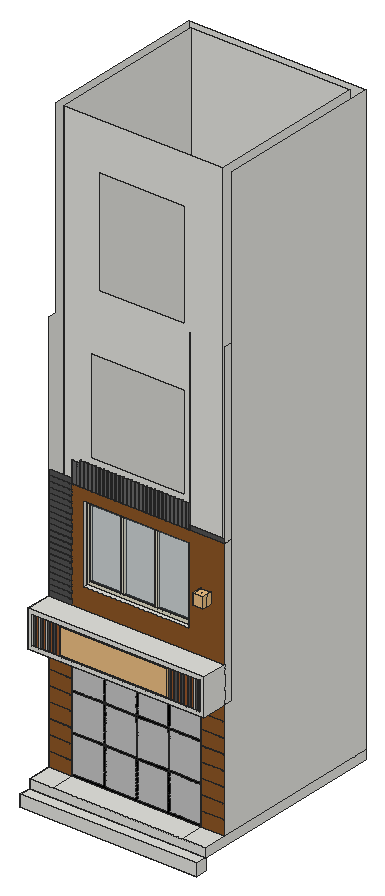
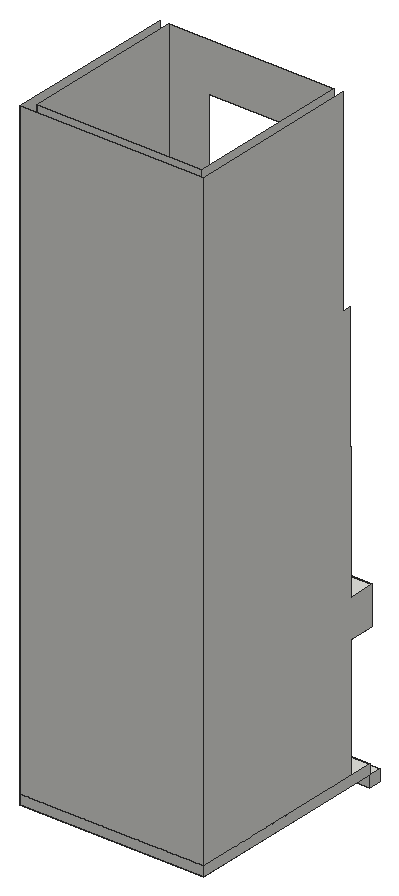
# SketchUp Ruby script. Lengths in inches.
U = 1.inch
M = Sketchup.active_model
def pt(a) = Geom::Point3d.new(a.map { |v| v * U })
def face(e, loops, mat)
  f = e.add_face(loops[0].map { |a| pt(a) })
  loops[1..].each { |l| e.add_face(l.map { |a| pt(a) }).erase! }
  f.material = f.back_material = mat if mat
  f
end
# faces: each face lists its corners as indices into pts; further lists are holes
def faces(e, pts, list, mat = nil) = list.each { |f| face(e, (f[0].is_a?(Array) ? f : [f]).map { |l| l.map { |i| pts[i] } }, mat) }
# xy, xz, yz: faces in a plane at the given z, y or x. An outline is a flat list of corners, or four numbers for a rectangle; further outlines are holes
def ring(l) = l.size == 4 ? [[l[0], l[1]], [l[2], l[1]], [l[2], l[3]], [l[0], l[3]]] : l.each_slice(2).to_a
def flat(e, list, mat, &to3) = list.each { |f| face(e, (f[0].is_a?(Array) ? f : [f]).map { |l| ring(l).map { |u, v| to3.(u, v) } }, mat) }
def xy(e, z, list, mat = nil) = flat(e, list, mat) { |x, y| [x, y, z] }
def xz(e, y, list, mat = nil) = flat(e, list, mat) { |x, z| [x, y, z] }
def yz(e, x, list, mat = nil) = flat(e, list, mat) { |y, z| [x, y, z] }
def lines(e, pts, list) = list.each { |a, b| e.add_line(pt(pts[a]), pt(pts[b])) }
# prism: a flat outline (further loops are holes) pulled along v
def prism(e, loops, v, mat = nil)
  f = face(e, loops, mat); d = Geom::Vector3d.new(v.map { |x| x * U })
  f.pushpull(f.normal.samedirection?(d) ? d.length : -d.length)
end
def box(e, o, s, mat = nil) = prism(e, [[o, [o[0] + s[0], o[1], o[2]], [o[0] + s[0], o[1] + s[1], o[2]], [o[0], o[1] + s[1], o[2]]]], [0, 0, s[2]], mat)
def at(x, y, z, deg = 0) = Geom::Transformation.translation(pt([x, y, z])) * Geom::Transformation.rotation(ORIGIN, Z_AXIS, deg.degrees)
def axes(o, x, y, z) = Geom::Transformation.new([*x, 0, *y, 0, *z, 0, *pt(o).to_a, 1])
def part(name) = M.definitions.add(name)
# library, detail: a bought-in or finely detailed component or shape, given as its bounding box
def library(name, o, s) = part(name).tap { |d| box(d.entities, o, s) }
def detail(e, o, s) = box(e.add_group.entities, o, s)
def put(e, d, t, mat = nil) = e.add_instance(d, t).tap { |i| i.material = mat if mat }
def group(e, t, mat = nil) = e.add_group.tap { |g| g.transformation = t; g.material = mat if mat }.entities
root = M.entities
M.materials.add("Glass").color = [171, 209, 242]
M.materials["Glass"].alpha = 0.09
M.materials.add("Plastic_SSS_01_White").color = [225, 221, 201]
M.materials.add("[0134_DimGray]").color = [105, 105, 105]
M.materials.add("[0135_DarkGray]").color = [81, 81, 81]
M.materials.add("[0137_Black]").color = [0, 0, 0]
M.materials.add("[Mirror 02]").color = [196, 196, 196]
M.materials.add("[Wood Cherry Original]").color = [152, 86, 42]
M.materials.add("[Wood Floor Dark]").color = [140, 86, 38]
c1 = library("JAIKOSH TRANING ",[0.06,0,0],[109.29,25.69,1])
c2 = part("Window frame")
xy(c2.entities,0,[[[104.47,83.98,176.47,131.98],[106.47,85.98,174.47,129.98]],[127.47,85.98,129.47,129.98],[150.47,85.98,152.47,129.98]],"Plastic_SSS_01_White")
xy(c2.entities,2,[[[104.47,83.98,176.47,131.98],[106.47,85.98,174.47,129.98]],[127.47,85.98,129.47,129.98],[150.47,85.98,152.47,129.98]],"Plastic_SSS_01_White")
xz(c2.entities,83.98,[[104.47,0,176.47,2]],"Plastic_SSS_01_White")
xz(c2.entities,85.98,[[106.47,0,127.47,2],[127.47,0,129.47,2],[129.47,0,150.47,2],[150.47,0,152.47,2],[152.47,0,174.47,2]],"Plastic_SSS_01_White")
xz(c2.entities,129.98,[[106.47,0,127.47,2],[127.47,0,129.47,2],[129.47,0,150.47,2],[150.47,0,152.47,2],[152.47,0,174.47,2]],"Plastic_SSS_01_White")
xz(c2.entities,131.98,[[104.47,0,176.47,2]],"Plastic_SSS_01_White")
yz(c2.entities,104.47,[[83.98,0,131.98,2]],"Plastic_SSS_01_White")
yz(c2.entities,106.47,[[85.98,0,129.98,2]],"Plastic_SSS_01_White")
yz(c2.entities,127.47,[[85.98,0,129.98,2]],"Plastic_SSS_01_White")
yz(c2.entities,129.47,[[85.98,0,129.98,2]],"Plastic_SSS_01_White")
yz(c2.entities,150.47,[[85.98,0,129.98,2]],"Plastic_SSS_01_White")
yz(c2.entities,152.47,[[85.98,0,129.98,2]],"Plastic_SSS_01_White")
yz(c2.entities,174.47,[[85.98,0,129.98,2]],"Plastic_SSS_01_White")
yz(c2.entities,176.47,[[83.98,0,131.98,2]],"Plastic_SSS_01_White")
c3 = part("Window pane")
box(c3.entities,[0,0,0],[67.88,44,0.5])
c4 = part("Glazed window assembly")
put(c4.entities,c2,at(-104.47,-83.98,0))
put(c4.entities,c3,at(2,2,0.7),"Glass")
c5 = part("window")
p = [[-596.28,88.12,20.39],[-668.28,88.12,20.39]]
lines(c5.entities,p,[[0,1]])
put(c5.entities,c4,axes([-668.28,88.12,20.39],[1,0,0],[0,0,1],[0,-1,0]))
c6 = library("Spot Light\#3",[-5.1,-5.1,-11.05],[10.2,10.2,11.05])
c7 = library("Spot Light\#2",[-5.1,-5.1,-11.05],[10.2,10.2,11.05])
xy(root,-21,[[0,11.5,180,23.5]])
xy(root,-9,[[0,11.5,180,23.5],[0,23.5,180,227.5]])
xy(root,0,[[0,23.5,24,47.5],[24,23.5,156,47.8125],[156,23.5,180,47.5],[[0,47.5,0,227.5,180,227.5,180,47.5,156,47.5,156,47.8125,24,47.8125,24,47.5],[9,56.5,171,218.5]],[9,56.5,171,218.5]])
xy(root,14.5,[[0,47.5,24,48],[156,47.5,180,48]])
xy(root,15,[[0,47.5,24,48],[156,47.5,180,48]])
xy(root,29.5,[[0,47.5,24,48],[156,47.5,180,48]])
xy(root,30,[[0,47.5,24,48],[156,47.5,180,48]])
xy(root,44.5,[[0,47.5,24,48],[156,47.5,180,48]])
xy(root,45,[[0,47.5,24,48],[156,47.5,180,48]])
xy(root,59.5,[[0,47.5,24,48],[156,47.5,180,47.8125]])
xy(root,60,[[0,47.5,24,48],[156,47.5,180,47.8125]])
xy(root,74.5,[[0,47.5,24,48],[156,47.5,180,48]])
xy(root,75,[[0,47.5,24,48],[156,47.5,180,48]])
xy(root,89.5,[[0,47.5,24,48],[156,47.5,180,48]])
xy(root,90,[[0,47.5,24,48],[156,47.5,180,48]])
xy(root,104.5,[[0,47.5,24,48],[156,47.5,180,48]])
xy(root,105,[[0,47.5,24,48],[156,47.5,180,48]])
xy(root,120,[[0,21.25,24,47.5],[24,21.25,156,47.8125],[156,21.25,180,47.5]])
xy(root,124,[[4,21.25,7.44,22.75],[7.44,21.25,10.88,22.25],[10.88,21.25,14.32,22.75],[14.32,21.25,17.76,22.5],[17.76,21.25,21.2,22.75],
  [21.2,21.25,24.64,22.5],[24.64,21.25,28.08,22.75],[28.08,21.25,31.52,22.5],[31.52,21.25,34.96,22.75],[34.96,21.25,38.4,22.375],
  [38.4,21.25,41.84,22.75],[41.84,21.25,45.28,22.5],[45.28,21.25,48.72,22.75],[48.72,21.25,52.16,22.5],[52.16,21.25,55.6,22.75],
  [55.6,21.25,59.04,22.5],[59.04,21.25,62.48,22.75],[62.48,21.25,65.92,22.5],[65.92,21.25,69.36,22.75],[69.36,21.25,72.8,22.5],
  [72.8,21.25,76.24,22.75],[76.24,21.25,79.68,22.5],[79.68,21.25,83.12,22.75],[83.12,21.25,86.56,22.5],[86.56,21.25,90,22.75],
  [90,21.25,93.44,22.5],[93.44,21.25,96.88,22.75],[96.88,21.25,100.32,22.5],[100.32,21.25,103.76,22.75],[103.76,21.25,107.2,22.5],
  [107.2,21.25,110.64,22.75],[110.64,21.25,114.08,22.5],[114.08,21.25,117.52,22.75],[117.52,21.25,120.96,22.5],[120.96,21.25,124.4,22.75],
  [124.4,21.25,127.84,22.5],[127.84,21.25,131.28,22.75],[131.28,21.25,134.72,22.5],[134.72,21.25,138.16,22.75],[138.16,21.25,141.6,22.5],
  [141.6,21.25,145.04,22.75],[145.04,21.25,148.48,22.5],[148.48,21.25,151.92,22.75],[151.92,21.25,155.36,22.5],[155.36,21.25,158.8,22.75],
  [158.8,21.25,162.24,22.5],[162.24,21.25,165.68,22.75],[165.68,21.25,169.12,22.5],[169.12,21.25,172.56,22.75],[172.56,21.25,176,22.5]])
xy(root,153,[[4,21.25,7.44,22.75],[7.44,21.25,10.88,22.25],[10.88,21.25,14.32,22.75],[14.32,21.25,17.76,22.5],[17.76,21.25,21.2,22.75],
  [21.2,21.25,24.64,22.5],[24.64,21.25,28.08,22.75],[28.08,21.25,31.52,22.5],[31.52,21.25,34.96,22.75],[34.96,21.25,38.4,22.375],
  [38.4,21.25,41.84,22.75],[41.84,21.25,45.28,22.5],[45.28,21.25,48.72,22.75],[48.72,21.25,52.16,22.5],[52.16,21.25,55.6,22.75],
  [55.6,21.25,59.04,22.5],[59.04,21.25,62.48,22.75],[62.48,21.25,65.92,22.5],[65.92,21.25,69.36,22.75],[69.36,21.25,72.8,22.5],
  [72.8,21.25,76.24,22.75],[76.24,21.25,79.68,22.5],[79.68,21.25,83.12,22.75],[83.12,21.25,86.56,22.5],[86.56,21.25,90,22.75],
  [90,21.25,93.44,22.5],[93.44,21.25,96.88,22.75],[96.88,21.25,100.32,22.5],[100.32,21.25,103.76,22.75],[103.76,21.25,107.2,22.5],
  [107.2,21.25,110.64,22.75],[110.64,21.25,114.08,22.5],[114.08,21.25,117.52,22.75],[117.52,21.25,120.96,22.5],[120.96,21.25,124.4,22.75],
  [124.4,21.25,127.84,22.5],[127.84,21.25,131.28,22.75],[131.28,21.25,134.72,22.5],[134.72,21.25,138.16,22.75],[138.16,21.25,141.6,22.5],
  [141.6,21.25,145.04,22.75],[145.04,21.25,148.48,22.5],[148.48,21.25,151.92,22.75],[151.92,21.25,155.36,22.5],[155.36,21.25,158.8,22.75],
  [158.8,21.25,162.24,22.5],[162.24,21.25,165.68,22.75],[165.68,21.25,169.12,22.5],[169.12,21.25,172.56,22.75],[172.56,21.25,176,22.5]])
xy(root,157,[[0,21.25,180,47.5]])
xy(root,162.05,[[0,47.5,24,48]])
xy(root,162.55,[[0,47.5,24,48]])
xy(root,167.6,[[0,47.5,24,48]])
xy(root,168.1,[[0,47.5,24,48]])
xy(root,173.15,[[0,47.5,24,48]])
xy(root,173.65,[[0,47.5,24,48]])
xy(root,178,[[36,47.5,144,56.5]])
xy(root,178.7,[[0,47.5,24,48]])
xy(root,179.2,[[0,47.5,24,48]])
xy(root,184.25,[[0,47.5,24,48]])
xy(root,184.75,[[0,47.5,24,48]])
xy(root,189.8,[[0,47.5,24,48]])
xy(root,190.3,[[0,47.5,24,48]])
xy(root,195.35,[[0,47.5,24,48]])
xy(root,195.85,[[0,47.5,24,48]])
xy(root,200.9,[[0,47.5,24,48]])
xy(root,201.4,[[0,47.5,24,48]])
xy(root,206.45,[[0,47.5,24,48]])
xy(root,206.95,[[0,47.5,24,48]])
xy(root,212,[[0,47.5,24,48]])
xy(root,212.5,[[0,47.5,24,48]])
xy(root,217.55,[[0,47.5,24,48]])
xy(root,218.05,[[0,47.5,24,48]])
xy(root,223.1,[[0,47.5,24,48]])
xy(root,223.6,[[0,47.5,24,48]])
xy(root,228.65,[[0,47.5,24,48]])
xy(root,229.15,[[0,47.5,24,48]])
xy(root,234.2,[[0,47.5,24,48]])
xy(root,234.7,[[0,47.5,24,48]])
xy(root,239.75,[[0,47.5,24,48]])
xy(root,240.25,[[0,47.5,24,48]])
xy(root,245.3,[[0,47.5,24,48]])
xy(root,245.8,[[0,47.5,24,48]])
xy(root,250.85,[[0,47.5,24,48]])
xy(root,251.35,[[0,47.5,24,48]])
xy(root,256,[[36,47.5,144,56.5]])
xy(root,256.4,[[0,47.5,24,48]])
xy(root,256.9,[[0,47.5,24,48]])
xy(root,261.95,[[0,47.5,24,48]])
xy(root,262.45,[[0,47.5,24,48]])
xy(root,267.45,[[0,47.5,24,48]],"[0135_DarkGray]")
xy(root,267.95,[[0,47.5,24,48]],"[0135_DarkGray]")
xy(root,268,[[24,47.5,24.5,48],[24.5,47.5,28,48],[28,47.5,28.5,48],[28.5,47.5,32,48],[32,47.5,32.5,48],
  [36,47.5,36.5,48],[40,47.5,40.5,48],[44,47.5,44.5,48],[48,47.5,48.5,48],[52,47.5,52.5,48],
  [56,47.5,56.5,48],[60,47.5,60.5,48],[64,47.5,64.5,48],[68,47.5,68.5,48],[72,47.5,72.5,48],
  [76,47.5,76.5,48],[80,47.5,80.5,48],[84,47.5,84.5,48],[88,47.5,88.5,48],[92,47.5,92.5,48],
  [96,47.5,96.5,48],[100,47.5,100.5,48],[104,47.5,104.5,48],[108,47.5,108.5,48],[112,47.5,112.5,48],
  [116,47.5,116.5,48],[120,47.5,120.5,48],[124,47.5,124.5,48],[128,47.5,128.5,48],[132,47.5,132.5,48],
  [136,47.5,136.5,48],[140,47.5,140.5,48],[144,47.5,144.5,48]],"[0135_DarkGray]")
xz(root,11.5,[[0,-21,180,-9]])
xz(root,21.25,[[[0,120,180,157],[4,124,176,153]]])
xz(root,22.25,[[7.44,124,10.88,153]],"[Wood Cherry Original]")
xz(root,22.375,[[34.96,124,38.4,153]],"[Wood Cherry Original]")
xz(root,22.5,[[14.32,124,17.76,153],[21.2,124,24.64,153],[28.08,124,31.52,153],[41.84,124,45.28,153],[48.72,124,52.16,153],
  [55.6,124,59.04,153],[62.48,124,65.92,153],[69.36,124,72.8,153],[76.24,124,79.68,153],[83.12,124,86.56,153],
  [90,124,93.44,153],[96.88,124,100.32,153],[103.76,124,107.2,153],[110.64,124,114.08,153],[117.52,124,120.96,153],
  [124.4,124,127.84,153],[131.28,124,134.72,153],[138.16,124,141.6,153],[145.04,124,148.48,153],[151.92,124,155.36,153],
  [158.8,124,162.24,153],[165.68,124,169.12,153],[172.56,124,176,153]],"[Wood Cherry Original]")
xz(root,22.75,[[4,124,7.44,153],[10.88,124,14.32,153],[17.76,124,21.2,153],[24.64,124,28.08,153],[31.52,124,34.96,153],
  [38.4,124,41.84,153],[45.28,124,48.72,153],[52.16,124,55.6,153],[59.04,124,62.48,153],[65.92,124,69.36,153],
  [72.8,124,76.24,153],[79.68,124,83.12,153],[86.56,124,90,153],[93.44,124,96.88,153],[100.32,124,103.76,153],
  [107.2,124,110.64,153],[114.08,124,117.52,153],[120.96,124,124.4,153],[127.84,124,131.28,153],[134.72,124,138.16,153],
  [141.6,124,145.04,153],[148.48,124,151.92,153],[155.36,124,158.8,153],[162.24,124,165.68,153],[169.12,124,172.56,153]],"[0135_DarkGray]")
xz(root,23.5,[[0,-21,180,-9],[0,-9,180,0]])
xz(root,47.5,[[32.5,268,36,292],[36.5,268,40,292],[40.5,268,44,292],[44.5,268,48,292],[48.5,268,52,292],
  [52.5,268,56,292],[56.5,268,60,292],[60.5,268,64,292],[64.5,268,68,292],[68.5,268,72,292],
  [72.5,268,76,292],[76.5,268,80,292],[80.5,268,84,292],[84.5,268,88,292],[88.5,268,92,292],
  [92.5,268,96,292],[96.5,268,100,292],[100.5,268,104,292],[104.5,268,108,292],[108.5,268,112,292],
  [112.5,268,116,292],[116.5,268,120,292],[120.5,268,124,292],[124.5,268,128,292],[128.5,268,132,292],
  [132.5,268,136,292],[136.5,268,140,292],[140.5,268,144,292]],"[0134_DimGray]")
xz(root,47.5,[[0,157,24,162.05],[0,162.55,24,167.6],[0,168.1,24,173.15],[0,173.65,24,178.7],[0,179.2,24,184.25],
  [0,184.75,24,189.8],[0,190.3,24,195.35],[0,195.85,24,200.9],[0,201.4,24,206.45],[0,206.95,24,212],
  [0,212.5,24,217.55],[0,218.05,24,223.1],[0,223.6,24,228.65],[0,229.15,24,234.2],[0,234.7,24,239.75],
  [0,240.25,24,245.3],[0,245.8,24,250.85],[0,251.35,24,256.4],[0,256.9,24,261.95],[0,262.45,24,267.45],
  [0,267.95,24,272.95],[144.5,268,180,272.3]],"[0135_DarkGray]")
xz(root,47.5,[[0,0,24,14.5],[156,0,180,14.5],[0,15,24,29.5],[156,15,180,29.5],[0,30,24,44.5],
  [156,30,180,44.5],[0,45,24,59.5],[156,45,180,59.5],[0,60,24,74.5],[156,60,180,74.5],
  [0,75,24,89.5],[156,75,180,89.5],[0,90,24,104.5],[156,90,180,104.5],[0,105,24,120],
  [156,105,180,120],[24,157,180,157,180,268,144,268,144,178,36,178,36,256,144,256,144,268,24,268]],"[Wood Floor Dark]")
xz(root,47.8125,[[24,0,156,0,156,2,124,2,124,38.67,122,38.67,122,2,91,2,91,38.67,89,38.67,89,2,58,2,58,38.67,56,38.67,56,2,24,2],[24,38.67,56,40.67],[56,38.67,58,40.67],[58,38.67,89,40.67],[89,38.67,91,40.67],
  [91,38.67,122,40.67],[122,38.67,124,40.67],[124,38.67,156,40.67],[56,40.67,58,77.33],[89,40.67,91,77.33],
  [122,40.67,124,77.33],[156,59.5,180,60],[24,77.33,56,79.33],[56,77.33,58,79.33],[58,77.33,89,79.33],
  [89,77.33,91,79.33],[91,77.33,122,79.33],[122,77.33,124,79.33],[124,77.33,156,79.33],[56,79.33,58,79.33,58,118,89,118,89,79.33,91,79.33,91,118,122,118,122,79.33,124,79.33,124,118,156,118,156,120,24,120,24,118,56,118]],"[0137_Black]")
xz(root,47.8125,[[24,2,56,38.67],[58,2,89,38.67],[91,2,122,38.67],[124,2,156,38.67],[24,40.67,56,77.33],
  [58,40.67,89,77.33],[91,40.67,122,77.33],[124,40.67,156,77.33],[24,79.33,56,118],[58,79.33,89,118],
  [91,79.33,122,118],[124,79.33,156,118]],"[Mirror 02]")
xz(root,48,[[24.5,268,28,289.45],[28.5,268,32,289.45]],"[0134_DimGray]")
xz(root,48,[[0,267.45,24,267.95]],"[0135_DarkGray]")
xz(root,48,[[0,14.5,24,15],[156,14.5,180,15],[0,29.5,24,30],[156,29.5,180,30],[0,44.5,24,45],
  [156,44.5,180,45],[0,59.5,24,60],[0,74.5,24,75],[156,74.5,180,75],[0,89.5,24,90],
  [156,89.5,180,90],[0,104.5,24,105],[156,104.5,180,105],[0,162.05,24,162.55],[0,167.6,24,168.1],
  [0,173.15,24,173.65],[0,178.7,24,179.2],[0,184.25,24,184.75],[0,189.8,24,190.3],[0,195.35,24,195.85],
  [0,200.9,24,201.4],[0,206.45,24,206.95],[0,212,24,212.5],[0,217.55,24,218.05],[0,223.1,24,223.6],
  [0,228.65,24,229.15],[0,234.2,24,234.7],[0,239.75,24,240.25],[0,245.3,24,245.8],[0,250.85,24,251.35],
  [0,256.4,24,256.9],[0,261.95,24,262.45],[24,268,24.5,289.45],[28,268,28.5,289.45],[32,268,32.5,289.45],
  [36,268,36.5,292],[40,268,40.5,292],[44,268,44.5,292],[48,268,48.5,292],[52,268,52.5,292],
  [56,268,56.5,292],[60,268,60.5,292],[64,268,64.5,292],[68,268,68.5,292],[72,268,72.5,292],
  [76,268,76.5,292],[80,268,80.5,292],[84,268,84.5,292],[88,268,88.5,292],[92,268,92.5,292],
  [96,268,96.5,292],[100,268,100.5,292],[104,268,104.5,292],[108,268,108.5,292],[112,268,112.5,292],
  [116,268,116.5,292],[120,268,120.5,292],[124,268,124.5,292],[128,268,128.5,292],[132,268,132.5,292],
  [136,268,136.5,292],[140,268,140.5,292],[144,268,144.5,268,144.5,448,143.6875,448,143.6875,412,144,292]],"[0137_Black]")
xz(root,56.5,[[[9,0,171,604.5],[44.8,448,132,556.5],[36,292,132,388],[36,178,144,256]]])
xz(root,218.5,[[9,0,171,604.5]])
xz(root,227.5,[[0,-9,180,0],[0,0,180,604.5]])
yz(root,0,[[11.5,-21,23.5,-9],[23.5,-9,227.5,0],[47.5,0,47.5,14.5,48,14.5,48,15,47.5,15,47.5,29.5,48,29.5,48,30,47.5,30,47.5,44.5,48,44.5,48,45,47.5,45,47.5,59.5,48,59.5,48,60,47.5,60,47.5,74.5,48,74.5,48,75,47.5,75,47.5,89.5,48,89.5,48,90,47.5,90,47.5,104.5,48,104.5,48,105,47.5,105,47.5,120,21.25,120,21.25,157,47.5,157,47.5,162.05,48,162.05,48,162.55,47.5,162.55,47.5,167.6,48,167.6,48,168.1,47.5,168.1,47.5,173.15,48,173.15,48,173.65,47.5,173.65,47.5,178.7,48,178.7,48,179.2,47.5,179.2,47.5,184.25,48,184.25,48,184.75,47.5,184.75,47.5,189.8,48,189.8,48,190.3,47.5,190.3,47.5,195.35,48,195.35,48,195.85,47.5,195.85,47.5,200.9,48,200.9,48,201.4,47.5,201.4,47.5,206.45,48,206.45,48,206.95,47.5,206.95,47.5,212,48,212,48,212.5,47.5,212.5,47.5,217.55,48,217.55,48,218.05,47.5,218.05,47.5,223.1,48,223.1,48,223.6,47.5,223.6,47.5,228.65,48,228.65,48,229.15,47.5,229.15,47.5,234.2,48,234.2,48,234.7,47.5,234.7,47.5,239.75,48,239.75,48,240.25,47.5,240.25,47.5,245.3,48,245.3,48,245.8,47.5,245.8,47.5,250.85,48,250.85,48,251.35,47.5,251.35,47.5,256.4,48,256.4,48,256.9,47.5,256.9,47.5,261.95,48,261.95,48,262.45,47.5,262.45,47.5,267.45,48,267.45,48,267.95,47.5,267.95,47.5,272.95,48,272.95,48,273.45,47.5,273.45,47.5,278.45,48,278.45,48,278.95,47.5,278.95,47.5,283.95,48,283.95,48,284.45,47.5,284.45,47.5,289.45,48,289.45,48,412,56.5,412,56.5,604.5,227.5,604.5,227.5,0]])
yz(root,4,[[21.25,124,22.75,153]])
yz(root,7.44,[[22.25,124,22.75,153]])
yz(root,9,[[56.5,0,218.5,604.5]])
yz(root,10.88,[[22.25,124,22.75,153]])
yz(root,14.32,[[22.5,124,22.75,153]])
yz(root,17.76,[[22.5,124,22.75,153]])
yz(root,21.2,[[22.5,124,22.75,153]])
yz(root,24,[[47.5,0,47.8125,14.5],[47.8125,14.5,48,15],[47.5,15,47.8125,29.5],[47.8125,29.5,48,30],[47.5,30,47.8125,44.5],
  [47.8125,44.5,48,45],[47.5,45,47.8125,59.5],[47.8125,59.5,48,60],[47.5,60,47.8125,74.5],[47.8125,74.5,48,75],
  [47.5,75,47.8125,89.5],[47.8125,89.5,48,90],[47.5,90,47.8125,104.5],[47.8125,104.5,48,105],[47.5,105,47.8125,120],
  [47.5,162.05,48,162.55],[47.5,167.6,48,168.1],[47.5,173.15,48,173.65],[47.5,178.7,48,179.2],[47.5,184.25,48,184.75],
  [47.5,189.8,48,190.3],[47.5,195.35,48,195.85],[47.5,200.9,48,201.4],[47.5,206.45,48,206.95],[47.5,212,48,212.5],
  [47.5,217.55,48,218.05],[47.5,223.1,48,223.6],[47.5,228.65,48,229.15],[47.5,234.2,48,234.7],[47.5,239.75,48,240.25],
  [47.5,245.3,48,245.8],[47.5,250.85,48,251.35],[47.5,256.4,48,256.9],[47.5,261.95,48,262.45]])
yz(root,24,[[47.5,267.45,48,267.95]],"[0135_DarkGray]")
yz(root,24,[[47.5,268,48,272.95]],"[0137_Black]")
yz(root,24.64,[[22.5,124,22.75,153]])
yz(root,28.08,[[22.5,124,22.75,153]])
yz(root,31.52,[[22.5,124,22.75,153]])
yz(root,32.5,[[47.5,268,48,292]],"[0135_DarkGray]")
yz(root,34.96,[[22.375,124,22.75,153]])
yz(root,36,[[47.5,178,56.5,256]])
yz(root,36,[[47.5,268,48,292]],"[0135_DarkGray]")
yz(root,36.5,[[47.5,268,48,292]],"[0135_DarkGray]")
yz(root,38.4,[[22.375,124,22.75,153]])
yz(root,40,[[47.5,268,48,292]],"[0135_DarkGray]")
yz(root,40.5,[[47.5,268,48,292]],"[0135_DarkGray]")
yz(root,41.84,[[22.5,124,22.75,153]])
yz(root,44,[[47.5,268,48,292]],"[0135_DarkGray]")
yz(root,44.5,[[47.5,268,48,292]],"[0135_DarkGray]")
yz(root,45.28,[[22.5,124,22.75,153]])
yz(root,48,[[47.5,268,48,292]],"[0135_DarkGray]")
yz(root,48.5,[[47.5,268,48,292]],"[0135_DarkGray]")
yz(root,48.72,[[22.5,124,22.75,153]])
yz(root,52,[[47.5,268,48,292]],"[0135_DarkGray]")
yz(root,52.16,[[22.5,124,22.75,153]])
yz(root,52.5,[[47.5,268,48,292]],"[0135_DarkGray]")
yz(root,55.6,[[22.5,124,22.75,153]])
yz(root,56,[[47.5,268,48,292]],"[0135_DarkGray]")
yz(root,56.5,[[47.5,268,48,292]],"[0135_DarkGray]")
yz(root,59.04,[[22.5,124,22.75,153]])
yz(root,60,[[47.5,268,48,292]],"[0135_DarkGray]")
yz(root,60.5,[[47.5,268,48,292]],"[0135_DarkGray]")
yz(root,62.48,[[22.5,124,22.75,153]])
yz(root,64,[[47.5,268,48,292]],"[0135_DarkGray]")
yz(root,64.5,[[47.5,268,48,292]],"[0135_DarkGray]")
yz(root,65.92,[[22.5,124,22.75,153]])
yz(root,68,[[47.5,268,48,292]],"[0135_DarkGray]")
yz(root,68.5,[[47.5,268,48,292]],"[0135_DarkGray]")
yz(root,69.36,[[22.5,124,22.75,153]])
yz(root,72,[[47.5,268,48,292]],"[0135_DarkGray]")
yz(root,72.5,[[47.5,268,48,292]],"[0135_DarkGray]")
yz(root,72.8,[[22.5,124,22.75,153]])
yz(root,76,[[47.5,268,48,292]],"[0135_DarkGray]")
yz(root,76.24,[[22.5,124,22.75,153]])
yz(root,76.5,[[47.5,268,48,292]],"[0135_DarkGray]")
yz(root,79.68,[[22.5,124,22.75,153]])
yz(root,80,[[47.5,268,48,292]],"[0135_DarkGray]")
yz(root,80.5,[[47.5,268,48,292]],"[0135_DarkGray]")
yz(root,83.12,[[22.5,124,22.75,153]])
yz(root,84,[[47.5,268,48,292]],"[0135_DarkGray]")
yz(root,84.5,[[47.5,268,48,292]],"[0135_DarkGray]")
yz(root,86.56,[[22.5,124,22.75,153]])
yz(root,88,[[47.5,268,48,292]],"[0135_DarkGray]")
yz(root,88.5,[[47.5,268,48,292]],"[0135_DarkGray]")
yz(root,90,[[22.5,124,22.75,153]])
yz(root,92,[[47.5,268,48,292]],"[0135_DarkGray]")
yz(root,92.5,[[47.5,268,48,292]],"[0135_DarkGray]")
yz(root,93.44,[[22.5,124,22.75,153]])
yz(root,96,[[47.5,268,48,292]],"[0135_DarkGray]")
yz(root,96.5,[[47.5,268,48,292]],"[0135_DarkGray]")
yz(root,96.88,[[22.5,124,22.75,153]])
yz(root,100,[[47.5,268,48,292]],"[0135_DarkGray]")
yz(root,100.32,[[22.5,124,22.75,153]])
yz(root,100.5,[[47.5,268,48,292]],"[0135_DarkGray]")
yz(root,103.76,[[22.5,124,22.75,153]])
yz(root,104,[[47.5,268,48,292]],"[0135_DarkGray]")
yz(root,104.5,[[47.5,268,48,292]],"[0135_DarkGray]")
yz(root,107.2,[[22.5,124,22.75,153]])
yz(root,108,[[47.5,268,48,292]],"[0135_DarkGray]")
yz(root,108.5,[[47.5,268,48,292]],"[0135_DarkGray]")
yz(root,110.64,[[22.5,124,22.75,153]])
yz(root,112,[[47.5,268,48,292]],"[0135_DarkGray]")
yz(root,112.5,[[47.5,268,48,292]],"[0135_DarkGray]")
yz(root,114.08,[[22.5,124,22.75,153]])
yz(root,116,[[47.5,268,48,292]],"[0135_DarkGray]")
yz(root,116.5,[[47.5,268,48,292]],"[0135_DarkGray]")
yz(root,117.52,[[22.5,124,22.75,153]])
yz(root,120,[[47.5,268,48,292]],"[0135_DarkGray]")
yz(root,120.5,[[47.5,268,48,292]],"[0135_DarkGray]")
yz(root,120.96,[[22.5,124,22.75,153]])
yz(root,124,[[47.5,268,48,292]],"[0135_DarkGray]")
yz(root,124.4,[[22.5,124,22.75,153]])
yz(root,124.5,[[47.5,268,48,292]],"[0135_DarkGray]")
yz(root,127.84,[[22.5,124,22.75,153]])
yz(root,128,[[47.5,268,48,292]],"[0135_DarkGray]")
yz(root,128.5,[[47.5,268,48,292]],"[0135_DarkGray]")
yz(root,131.28,[[22.5,124,22.75,153]])
yz(root,132,[[47.5,268,48,292]],"[0135_DarkGray]")
yz(root,132.5,[[47.5,268,48,292]],"[0135_DarkGray]")
yz(root,134.72,[[22.5,124,22.75,153]])
yz(root,136,[[47.5,268,48,292]],"[0135_DarkGray]")
yz(root,136.5,[[47.5,268,48,292]],"[0135_DarkGray]")
yz(root,138.16,[[22.5,124,22.75,153]])
yz(root,140,[[47.5,268,48,292]],"[0135_DarkGray]")
yz(root,140.5,[[47.5,268,48,292]],"[0135_DarkGray]")
yz(root,141.6,[[22.5,124,22.75,153]])
yz(root,144,[[47.5,178,56.5,256]])
yz(root,144,[[47.5,268,48,292]],"[0135_DarkGray]")
yz(root,144.5,[[47.5,268,48,272.3]],"[0135_DarkGray]")
yz(root,145.04,[[22.5,124,22.75,153]])
yz(root,148.48,[[22.5,124,22.75,153]])
yz(root,151.92,[[22.5,124,22.75,153]])
yz(root,155.36,[[22.5,124,22.75,153]])
yz(root,156,[[47.5,0,47.8125,14.5],[47.8125,14.5,48,15],[47.5,15,47.8125,29.5],[47.8125,29.5,48,30],[47.5,30,47.8125,44.5],
  [47.8125,44.5,48,45],[47.5,45,47.8125,59.5],[47.5,60,47.8125,74.5],[47.8125,74.5,48,75],[47.5,75,47.8125,89.5],
  [47.8125,89.5,48,90],[47.5,90,47.8125,104.5],[47.8125,104.5,48,105],[47.5,105,47.8125,120]])
yz(root,158.8,[[22.5,124,22.75,153]])
yz(root,162.24,[[22.5,124,22.75,153]])
yz(root,165.68,[[22.5,124,22.75,153]])
yz(root,169.12,[[22.5,124,22.75,153]])
yz(root,171,[[56.5,0,218.5,604.5]])
yz(root,172.56,[[22.5,124,22.75,153]])
yz(root,176,[[21.25,124,22.5,153]])
yz(root,180,[[11.5,-21,23.5,-9],[23.5,-9,227.5,0],[47.5,0,227.5,0,227.5,604.5,56.5,604.5,56.5,120,47.5,120,47.5,105,48,105,48,104.5,47.5,104.5,47.5,90,48,90,48,89.5,47.5,89.5,47.5,75,48,75,48,74.5,47.5,74.5,47.5,60,47.8125,60,47.8125,59.5,47.5,59.5,47.5,45,48,45,48,44.5,47.5,44.5,47.5,30,48,30,48,29.5,47.5,29.5,47.5,15,48,15,48,14.5,47.5,14.5],[21.25,120,47.5,157],[47.5,120,56.5,268],
  [47.5,268,56.5,268,56.5,448,47.5,448,47.5,407.2,48,407.2,48,406.7,47.5,406.7,47.5,402.4,48,402.4,48,401.9,47.5,401.9,47.5,397.6,48,397.6,48,397.1,47.5,397.1,47.5,392.8,48,392.8,48,392.3,47.5,392.3,47.5,388,48,388,48,387.5,47.5,387.5,47.5,383.2,48,383.2,48,382.7,47.5,382.7,47.5,378.4,48,378.4,48,377.9,47.5,377.9,47.5,373.6,48,373.6,48,373.1,47.5,373.1,47.5,368.8,48,368.8,48,368.3,47.5,368.3,47.5,364,48,364,48,363.5,47.5,363.5,47.5,359.2,48,359.2,48,358.7,47.5,358.7,47.5,354.4,48,354.4,48,353.9,47.5,353.9,47.5,349.6,48,349.6,48,349.1,47.5,349.1,47.5,344.8,48,344.8,48,344.3,47.5,344.3,47.5,340,48,340,48,339.5,47.5,339.5,47.5,335.2,48,335.2,48,334.7,47.5,334.7,47.5,330.4,48,330.4,48,329.9,47.5,329.9,47.5,325.6,48,325.6,48,325.1,47.5,325.1,47.5,320.8,48,320.8,48,320.3,47.5,320.3,47.5,316,48,316,48,315.5,47.5,315.5,47.5,311.2,48,311.2,48,310.7,47.5,310.7,47.5,306.4,48,306.4,48,305.9,47.5,305.9,47.5,301.6,48,301.6,48,301.1,47.5,301.1,47.5,296.8,48,296.8,48,296.3,47.5,296.3,47.5,292,48,292,48,291.5,47.5,291.5,47.5,287.2,48,287.2,48,286.7,47.5,286.7,47.5,282.4,48,282.4,48,281.9,47.5,281.9,47.5,277.6,48,277.6,48,277.1,47.5,277.1,47.5,272.8,48,272.8,48,272.3,47.5,272.3]])
p = [[24,48.125,2],[56,48.125,2]]
lines(root,p,[[0,1]])
put(root,c1,axes([33.82,21.25,126.14],[1,0,0],[0,0,1],[0,-1,0]))
put(root,c5,axes([1038.43,-34.12,144.86],[1.5,0,0],[0,1,0],[0,0,1.625]))
put(root,c6,at(161.08,47.5,218.45))
put(root,c7,at(161.08,42.4,218.46))
